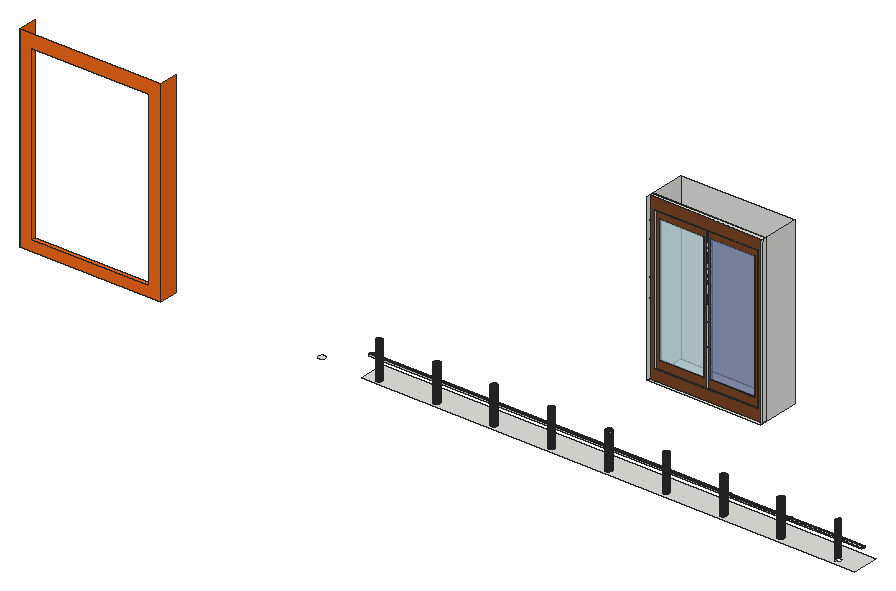
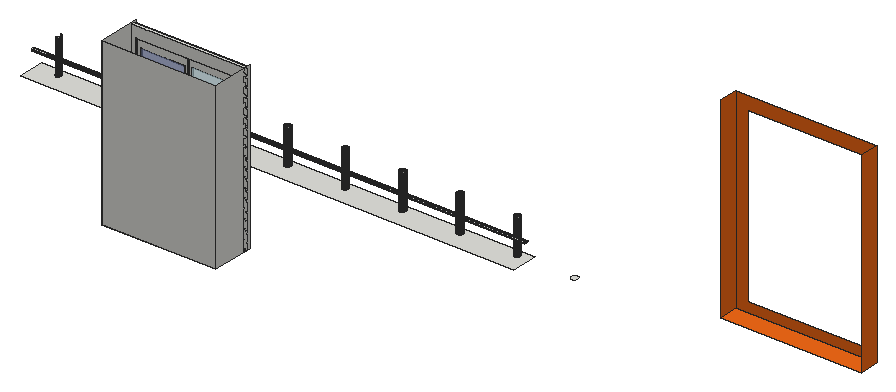
# SketchUp Ruby script. Lengths in inches.
U = 1.inch
M = Sketchup.active_model
def pt(a) = Geom::Point3d.new(a.map { |v| v * U })
def face(e, loops, mat)
  f = e.add_face(loops[0].map { |a| pt(a) })
  loops[1..].each { |l| e.add_face(l.map { |a| pt(a) }).erase! }
  f.material = f.back_material = mat if mat
  f
end
# faces: each face lists its corners as indices into pts; further lists are holes
def faces(e, pts, list, mat = nil) = list.each { |f| face(e, (f[0].is_a?(Array) ? f : [f]).map { |l| l.map { |i| pts[i] } }, mat) }
# xy, xz, yz: faces in a plane at the given z, y or x. An outline is a flat list of corners, or four numbers for a rectangle; further outlines are holes
def ring(l) = l.size == 4 ? [[l[0], l[1]], [l[2], l[1]], [l[2], l[3]], [l[0], l[3]]] : l.each_slice(2).to_a
def flat(e, list, mat, &to3) = list.each { |f| face(e, (f[0].is_a?(Array) ? f : [f]).map { |l| ring(l).map { |u, v| to3.(u, v) } }, mat) }
def xy(e, z, list, mat = nil) = flat(e, list, mat) { |x, y| [x, y, z] }
def xz(e, y, list, mat = nil) = flat(e, list, mat) { |x, z| [x, y, z] }
def yz(e, x, list, mat = nil) = flat(e, list, mat) { |y, z| [x, y, z] }
def lines(e, pts, list) = list.each { |a, b| e.add_line(pt(pts[a]), pt(pts[b])) }
# prism: a flat outline (further loops are holes) pulled along v
def prism(e, loops, v, mat = nil)
  f = face(e, loops, mat); d = Geom::Vector3d.new(v.map { |x| x * U })
  f.pushpull(f.normal.samedirection?(d) ? d.length : -d.length)
end
def box(e, o, s, mat = nil) = prism(e, [[o, [o[0] + s[0], o[1], o[2]], [o[0] + s[0], o[1] + s[1], o[2]], [o[0], o[1] + s[1], o[2]]]], [0, 0, s[2]], mat)
def at(x, y, z, deg = 0) = Geom::Transformation.translation(pt([x, y, z])) * Geom::Transformation.rotation(ORIGIN, Z_AXIS, deg.degrees)
def axes(o, x, y, z) = Geom::Transformation.new([*x, 0, *y, 0, *z, 0, *pt(o).to_a, 1])
def part(name) = M.definitions.add(name)
# library, detail: a bought-in or finely detailed component or shape, given as its bounding box
def library(name, o, s) = part(name).tap { |d| box(d.entities, o, s) }
def detail(e, o, s) = box(e.add_group.entities, o, s)
def put(e, d, t, mat = nil) = e.add_instance(d, t).tap { |i| i.material = mat if mat }
def group(e, t, mat = nil) = e.add_group.tap { |g| g.transformation = t; g.material = mat if mat }.entities
root = M.entities
M.materials.add("Generic").color = [243, 106, 23]
M.materials.add("[Translucent_Glass_Safety]").color = [204, 235, 244]
M.materials["[Translucent_Glass_Safety]"].alpha = 0.5
M.materials.add("[Translucent_Glass_Sky_Reflection]").color = [125, 138, 183]
M.materials["[Translucent_Glass_Sky_Reflection]"].alpha = 0.52
M.materials.add("[Wood Veneer 01]").color = [120, 70, 37]
c1 = part("Sliding window")
xy(c1.entities,0,[[0,0,4.33,55.51]])
xy(c1.entities,2.76,[[0,2.76,2,27.76],[3.15,2.76,4.33,27.76],[0,27.76,0.82,52.76],[0.82,27.76,2.36,52.76],[2.36,27.76,4.33,52.76]])
xy(c1.entities,4.72,[[2,4.72,2.4,26.38],[2.76,4.72,3.15,26.38],[0.82,29.13,1.22,50.79],[1.97,29.13,2.36,50.79]])
xy(c1.entities,36.61,[[2,4.72,2.4,26.38],[2.76,4.72,3.15,26.38],[0.82,29.13,1.22,50.79],[1.97,29.13,2.36,50.79]])
xy(c1.entities,38.58,[[0,2.76,2,27.76],[3.15,2.76,4.33,27.76],[0,27.76,0.82,52.76],[0.82,27.76,2.36,52.76],[2.36,27.76,4.33,52.76]])
xy(c1.entities,41.34,[[0,0,4.33,55.51]])
xz(c1.entities,0,[[0,0,4.33,41.34]])
xz(c1.entities,2.76,[[0,2.76,2,38.58],[3.15,2.76,4.33,38.58]])
xz(c1.entities,4.72,[[2,4.72,2.4,36.61],[2.76,4.72,3.15,36.61]])
xz(c1.entities,26.38,[[2,4.72,2.4,36.61],[2.76,4.72,3.15,36.61]])
xz(c1.entities,27.76,[[0.82,2.76,2,38.58],[2,2.76,2.36,38.58],[2.36,2.76,3.15,38.58]])
xz(c1.entities,29.13,[[0.82,4.72,1.22,36.61],[1.97,4.72,2.36,36.61]])
xz(c1.entities,50.79,[[0.82,4.72,1.22,36.61],[1.97,4.72,2.36,36.61]])
xz(c1.entities,52.76,[[0,2.76,0.82,38.58],[0.82,2.76,2.36,38.58],[2.36,2.76,4.33,38.58]])
xz(c1.entities,55.51,[[0,0,4.33,41.34]])
yz(c1.entities,0,[[[0,0,55.51,41.34],[2.76,2.76,52.76,38.58]]])
yz(c1.entities,0.82,[[[27.76,2.76,52.76,38.58],[29.13,4.72,50.79,36.61]]])
yz(c1.entities,1.22,[[29.13,4.72,50.79,36.61]],"[Translucent_Glass_Sky_Reflection]")
yz(c1.entities,1.97,[[29.13,4.72,50.79,36.61]],"[Translucent_Glass_Sky_Reflection]")
yz(c1.entities,2,[[[2.76,2.76,27.76,38.58],[4.72,4.72,26.38,36.61]]])
yz(c1.entities,2.36,[[[27.76,2.76,52.76,38.58],[29.13,4.72,50.79,36.61]]],"[Wood Veneer 01]")
yz(c1.entities,2.4,[[4.72,4.72,26.38,36.61]],"[Translucent_Glass_Safety]")
yz(c1.entities,2.76,[[4.72,4.72,26.38,36.61]],"[Translucent_Glass_Safety]")
yz(c1.entities,3.15,[[[2.76,2.76,27.76,38.58],[4.72,4.72,26.38,36.61]]],"[Wood Veneer 01]")
yz(c1.entities,4.33,[[[0,0,55.51,41.34],[2.76,2.76,52.76,38.58]]],"[Wood Veneer 01]")
xy(root,143.28,[[[220.54,127.4375,383.85,136.1875],[338.54,128.64,338.28,128.68,338.04,128.78,337.83,128.9375,337.67,129.14,337.57,129.39,337.54,129.64,337.57,129.9,337.67,130.14,337.83,130.35,338.04,130.51,338.28,130.61,338.54,130.64,338.79,130.61,339.04,130.51,339.24,130.35,339.4,130.14,339.5,129.9,339.54,129.64,339.5,129.39,339.4,129.14,339.24,128.9375,339.04,128.78,338.79,128.68],[319.54,128.64,319.28,128.68,319.04,128.78,318.83,128.9375,318.67,129.14,318.57,129.39,318.54,129.64,318.57,129.9,318.67,130.14,318.83,130.35,319.04,130.51,319.28,130.61,319.54,130.64,319.79,130.61,320.04,130.51,320.24,130.35,320.4,130.14,320.5,129.9,320.54,129.64,320.5,129.39,320.4,129.14,320.24,128.9375,320.04,128.78,319.79,128.68],[300.54,128.64,300.28,128.68,300.04,128.78,299.83,128.9375,299.67,129.14,299.57,129.39,299.54,129.64,299.57,129.9,299.67,130.14,299.83,130.35,300.04,130.51,300.28,130.61,300.54,130.64,300.79,130.61,301.04,130.51,301.24,130.35,301.4,130.14,301.5,129.9,301.54,129.64,301.5,129.39,301.4,129.14,301.24,128.9375,301.04,128.78,300.79,128.68],[281.54,128.64,281.28,128.68,281.04,128.78,280.83,128.9375,280.67,129.14,280.57,129.39,280.54,129.64,280.57,129.9,280.67,130.14,280.83,130.35,281.04,130.51,281.28,130.61,281.54,130.64,281.79,130.61,282.04,130.51,282.24,130.35,282.4,130.14,282.5,129.9,282.54,129.64,282.5,129.39,282.4,129.14,282.24,128.9375,282.04,128.78,281.79,128.68],[262.54,128.64,262.28,128.68,262.04,128.78,261.83,128.9375,261.67,129.14,261.57,129.39,261.54,129.64,261.57,129.9,261.67,130.14,261.83,130.35,262.04,130.51,262.28,130.61,262.54,130.64,262.79,130.61,263.04,130.51,263.24,130.35,263.4,130.14,263.5,129.9,263.54,129.64,263.5,129.39,263.4,129.14,263.24,128.9375,263.04,128.78,262.79,128.68],[243.54,128.64,243.28,128.68,243.04,128.78,242.83,128.9375,242.67,129.14,242.57,129.39,242.54,129.64,242.57,129.9,242.67,130.14,242.83,130.35,243.04,130.51,243.28,130.61,243.54,130.64,243.79,130.61,244.04,130.51,244.24,130.35,244.4,130.14,244.5,129.9,244.54,129.64,244.5,129.39,244.4,129.14,244.24,128.9375,244.04,128.78,243.79,128.68],[224.54,128.64,224.28,128.68,224.04,128.78,223.83,128.9375,223.67,129.14,223.57,129.39,223.54,129.64,223.57,129.9,223.67,130.14,223.83,130.35,224.04,130.51,224.28,130.61,224.54,130.64,224.79,130.61,225.04,130.51,225.24,130.35,225.4,130.14,225.5,129.9,225.54,129.64,225.5,129.39,225.4,129.14,225.24,128.9375,225.04,128.78,224.79,128.68],[376.66,128.64,376.4,128.68,376.16,128.78,375.95,128.9375,375.79,129.14,375.69,129.39,375.66,129.64,375.69,129.9,375.79,130.14,375.95,130.35,376.16,130.51,376.4,130.61,376.66,130.64,376.92,130.61,377.16,130.51,377.37,130.35,377.53,130.14,377.625,129.9,377.66,129.64,377.625,129.39,377.53,129.14,377.37,128.9375,377.16,128.78,376.92,128.68],[357.54,128.64,357.28,128.68,357.04,128.78,356.83,128.9375,356.67,129.14,356.57,129.39,356.54,129.64,356.57,129.9,356.67,130.14,356.83,130.35,357.04,130.51,357.28,130.61,357.54,130.64,357.79,130.61,358.04,130.51,358.24,130.35,358.4,130.14,358.5,129.9,358.54,129.64,358.5,129.39,358.4,129.14,358.24,128.9375,358.04,128.78,357.79,128.68]],[205.54,128.64,205.79,128.68,206.04,128.78,206.24,128.9375,206.4,129.14,206.5,129.39,206.54,129.64,206.5,129.9,206.4,130.14,206.24,130.35,206.04,130.51,205.79,130.61,205.54,130.64,205.28,130.61,205.04,130.51,204.83,130.35,204.67,130.14,204.57,129.9,204.54,129.64,204.57,129.39,204.67,129.14,204.83,128.9375,205.04,128.78,205.28,128.68]])
xy(root,144.25,[[279.74,171.4375,317.36,185.375]])
xy(root,146.92,[[112.41,121.25,158.88,127.4375]],"Generic")
xy(root,148.75,[[220.54,130.19,320.53,130.82],[320.53,130.19,338.84,130.82],[338.84,130.19,359.16,130.82],[359.16,130.19,378.85,130.82]])
xy(root,149.1875,[[220.54,130.19,320.53,130.82],[320.53,130.19,338.84,130.82],[338.84,130.19,383.85,130.82]])
xz(root,121.25,[[[112.41,146.92,158.88,211.52],[115.79,150.18,154.87,207.14]]],"Generic")
xz(root,130.19,[[220.54,148.75,383.85,149.1875]])
xz(root,130.82,[[220.54,149.0625,320.53,149.1875],[220.54,149.0625,320.53,149.1875],[320.53,149.0625,338.84,149.1875],[320.53,149.0625,338.84,149.1875],[338.84,149.0625,359.16,149.1875],
  [338.84,149.0625,359.16,149.1875],[359.16,149.0625,378.85,149.1875],[359.16,149.0625,378.85,149.1875]])
xz(root,131.35,[[220.54,148.72,383.85,149.04]])
xz(root,185.375,[[279.74,144.25,317.36,198.6875]])
yz(root,112.41,[[121.25,146.92,127.4375,211.52]],"Generic")
yz(root,158.88,[[121.25,146.92,127.4375,211.52]],"Generic")
yz(root,279.74,[[171.4375,144.25,185.375,198.6875]])
yz(root,317.36,[[171.4375,144.25,185.375,198.6875]])
p = [[224.28,128.68,143.28],[224.54,128.64,143.28],[224.54,128.64,155.04],[224.28,128.68,155.04],[224.79,128.68,143.28],[224.79,128.68,155.04],
  [243.28,128.68,143.28],[243.54,128.64,143.28],[243.54,128.64,155.04],[243.28,128.68,155.04],[243.79,128.68,143.28],[243.79,128.68,155.04],
  [262.28,128.68,143.28],[262.54,128.64,143.28],[262.54,128.64,155.04],[262.28,128.68,155.04],[262.79,128.68,143.28],[262.79,128.68,155.04],
  [281.28,128.68,143.28],[281.54,128.64,143.28],[281.54,128.64,155.04],[281.28,128.68,155.04],[281.79,128.68,143.28],[281.79,128.68,155.04],
  [300.28,128.68,143.28],[300.54,128.64,143.28],[300.54,128.64,155.04],[300.28,128.68,155.04],[300.79,128.68,143.28],[300.79,128.68,155.04],
  [319.28,128.68,143.28],[319.54,128.64,143.28],[319.54,128.64,155.04],[319.28,128.68,155.04],[319.79,128.68,143.28],[319.79,128.68,155.04],
  [338.28,128.68,143.28],[338.54,128.64,143.28],[338.54,128.64,155.04],[338.28,128.68,155.04],[338.79,128.68,143.28],[338.79,128.68,155.04],
  [357.28,128.68,143.28],[357.54,128.64,143.28],[357.54,128.64,155.04],[357.28,128.68,155.04],[357.79,128.68,143.28],[357.79,128.68,155.04],
  [224.04,128.78,143.28],[224.04,128.78,155.04],[225.04,128.78,143.28],[225.04,128.78,155.04],[243.04,128.78,143.28],[243.04,128.78,155.04],
  [244.04,128.78,143.28],[244.04,128.78,155.04],[262.04,128.78,143.28],[262.04,128.78,155.04],[263.04,128.78,143.28],[263.04,128.78,155.04],
  [281.04,128.78,143.28],[281.04,128.78,155.04],[282.04,128.78,143.28],[282.04,128.78,155.04],[300.04,128.78,143.28],[300.04,128.78,155.04],
  [301.04,128.78,143.28],[301.04,128.78,155.04],[319.04,128.78,143.28],[319.04,128.78,155.04],[320.04,128.78,143.28],[320.04,128.78,155.04],
  [338.04,128.78,143.28],[338.04,128.78,155.04],[339.04,128.78,143.28],[339.04,128.78,155.04],[357.04,128.78,143.28],[357.04,128.78,155.04],
  [358.04,128.78,143.28],[358.04,128.78,155.04],[376.16,128.78,143.28],[376.4,128.68,143.28],[376.4,128.68,155.04],[376.16,128.78,155.04],
  [223.83,128.9375,143.28],[223.83,128.9375,155.04],[225.24,128.9375,143.28],[225.24,128.9375,155.04],[242.83,128.9375,143.28],[242.83,128.9375,155.04],
  [244.24,128.9375,143.28],[244.24,128.9375,155.04],[261.83,128.9375,143.28],[261.83,128.9375,155.04],[263.24,128.9375,143.28],[263.24,128.9375,155.04],
  [280.83,128.9375,143.28],[280.83,128.9375,155.04],[282.24,128.9375,143.28],[282.24,128.9375,155.04],[299.83,128.9375,143.28],[299.83,128.9375,155.04],
  [301.24,128.9375,143.28],[301.24,128.9375,155.04],[318.83,128.9375,143.28],[318.83,128.9375,155.04],[320.24,128.9375,143.28],[320.24,128.9375,155.04],
  [337.83,128.9375,143.28],[337.83,128.9375,155.04],[339.24,128.9375,143.28],[339.24,128.9375,155.04],[356.83,128.9375,143.28],[356.83,128.9375,155.04],
  [358.24,128.9375,143.28],[358.24,128.9375,155.04],[375.95,128.9375,143.28],[375.95,128.9375,155.04],[223.67,129.14,143.28],[223.67,129.14,155.04],
  [225.4,129.14,143.28],[225.4,129.14,155.04],[242.67,129.14,143.28],[242.67,129.14,155.04],[244.4,129.14,143.28],[244.4,129.14,155.04],
  [261.67,129.14,143.28],[261.67,129.14,155.04],[263.4,129.14,143.28],[263.4,129.14,155.04],[280.67,129.14,143.28],[280.67,129.14,155.04],
  [282.4,129.14,143.28],[282.4,129.14,155.04],[299.67,129.14,143.28],[299.67,129.14,155.04],[301.4,129.14,143.28],[301.4,129.14,155.04],
  [318.67,129.14,143.28],[318.67,129.14,155.04],[320.4,129.14,143.28],[320.4,129.14,155.04],[337.67,129.14,143.28],[337.67,129.14,155.04],
  [339.4,129.14,143.28],[339.4,129.14,155.04],[356.67,129.14,143.28],[356.67,129.14,155.04],[358.4,129.14,143.28],[358.4,129.14,155.04],
  [375.79,129.14,143.28],[375.79,129.14,155.04],[223.57,129.39,143.28],[223.57,129.39,155.04],[225.5,129.39,143.28],[225.5,129.39,155.04],
  [242.57,129.39,143.28],[242.57,129.39,155.04],[244.5,129.39,143.28],[244.5,129.39,155.04],[261.57,129.39,143.28],[261.57,129.39,155.04],
  [263.5,129.39,143.28],[263.5,129.39,155.04],[280.57,129.39,143.28],[280.57,129.39,155.04],[282.5,129.39,143.28],[282.5,129.39,155.04],
  [299.57,129.39,143.28],[299.57,129.39,155.04],[301.5,129.39,143.28],[301.5,129.39,155.04],[318.57,129.39,143.28],[318.57,129.39,155.04],
  [320.5,129.39,143.28],[320.5,129.39,155.04],[337.57,129.39,143.28],[337.57,129.39,155.04],[339.5,129.39,143.28],[339.5,129.39,155.04],
  [356.57,129.39,143.28],[356.57,129.39,155.04],[358.5,129.39,143.28],[358.5,129.39,155.04],[375.69,129.39,143.28],[375.69,129.39,155.04],
  [223.54,129.64,143.28],[223.54,129.64,155.04],[225.54,129.64,143.28],[225.54,129.64,155.04],[242.54,129.64,143.28],[242.54,129.64,155.04],
  [244.54,129.64,143.28],[244.54,129.64,155.04],[261.54,129.64,143.28],[261.54,129.64,155.04],[263.54,129.64,143.28],[263.54,129.64,155.04],
  [280.54,129.64,143.28],[280.54,129.64,155.04],[282.54,129.64,143.28],[282.54,129.64,155.04],[299.54,129.64,143.28],[299.54,129.64,155.04],
  [301.54,129.64,143.28],[301.54,129.64,155.04],[318.54,129.64,143.28],[318.54,129.64,155.04],[320.54,129.64,143.28],[320.54,129.64,155.04],
  [337.54,129.64,143.28],[337.54,129.64,155.04],[339.54,129.64,143.28],[339.54,129.64,155.04],[356.54,129.64,143.28],[356.54,129.64,155.04],
  [358.54,129.64,143.28],[358.54,129.64,155.04],[375.66,129.64,143.28],[375.66,129.64,155.04],[223.57,129.9,143.28],[223.57,129.9,155.04],
  [225.5,129.9,143.28],[225.5,129.9,155.04],[242.57,129.9,143.28],[242.57,129.9,155.04],[244.5,129.9,143.28],[244.5,129.9,155.04],
  [261.57,129.9,143.28],[261.57,129.9,155.04],[263.5,129.9,143.28],[263.5,129.9,155.04],[280.57,129.9,143.28],[280.57,129.9,155.04],
  [282.5,129.9,143.28],[282.5,129.9,155.04],[299.57,129.9,143.28],[299.57,129.9,155.04],[301.5,129.9,143.28],[301.5,129.9,155.04],
  [318.57,129.9,143.28],[318.57,129.9,155.04],[320.5,129.9,143.28],[320.5,129.9,155.04],[337.57,129.9,143.28],[337.57,129.9,155.04],
  [339.5,129.9,143.28],[339.5,129.9,155.04],[356.57,129.9,143.28],[356.57,129.9,155.04],[358.5,129.9,143.28],[358.5,129.9,155.04],
  [375.69,129.9,143.28],[375.69,129.9,155.04],[223.67,130.14,143.28],[223.67,130.14,155.04],[225.4,130.14,143.28],[225.4,130.14,155.04],
  [242.67,130.14,143.28],[242.67,130.14,155.04],[244.4,130.14,143.28],[244.4,130.14,155.04],[261.67,130.14,143.28],[261.67,130.14,155.04],
  [263.4,130.14,143.28],[263.4,130.14,155.04],[280.67,130.14,143.28],[280.67,130.14,155.04],[282.4,130.14,143.28],[282.4,130.14,155.04],
  [299.67,130.14,143.28],[299.67,130.14,155.04],[301.4,130.14,143.28],[301.4,130.14,155.04],[318.67,130.14,143.28],[318.67,130.14,155.04],
  [320.4,130.14,143.28],[320.4,130.14,155.04],[337.67,130.14,143.28],[337.67,130.14,155.04],[339.4,130.14,143.28],[339.4,130.14,155.04],
  [356.67,130.14,143.28],[356.67,130.14,155.04],[358.4,130.14,143.28],[358.4,130.14,155.04],[375.79,130.14,143.28],[375.79,130.14,155.04],
  [223.83,130.35,143.28],[223.83,130.35,155.04],[225.24,130.35,143.28],[225.24,130.35,155.04],[242.83,130.35,143.28],[242.83,130.35,155.04],
  [244.24,130.35,143.28],[244.24,130.35,155.04],[261.83,130.35,143.28],[261.83,130.35,155.04],[263.24,130.35,143.28],[263.24,130.35,155.04],
  [280.83,130.35,143.28],[280.83,130.35,155.04],[282.24,130.35,143.28],[282.24,130.35,155.04],[299.83,130.35,143.28],[299.83,130.35,155.04],
  [301.24,130.35,143.28],[301.24,130.35,155.04],[318.83,130.35,143.28],[318.83,130.35,155.04],[320.24,130.35,143.28],[320.24,130.35,155.04],
  [337.83,130.35,143.28],[337.83,130.35,155.04],[339.24,130.35,143.28],[339.24,130.35,155.04],[356.83,130.35,143.28],[356.83,130.35,155.04],
  [358.24,130.35,143.28],[358.24,130.35,155.04],[375.95,130.35,143.28],[375.95,130.35,155.04],[224.04,130.51,143.28],[224.04,130.51,155.04],
  [225.04,130.51,143.28],[225.04,130.51,155.04],[243.04,130.51,143.28],[243.04,130.51,155.04],[244.04,130.51,143.28],[244.04,130.51,155.04],
  [262.04,130.51,143.28],[262.04,130.51,155.04],[263.04,130.51,143.28],[263.04,130.51,155.04],[281.04,130.51,143.28],[281.04,130.51,155.04],
  [282.04,130.51,143.28],[282.04,130.51,155.04],[300.04,130.51,143.28],[300.04,130.51,155.04],[301.04,130.51,143.28],[301.04,130.51,155.04],
  [319.04,130.51,143.28],[319.04,130.51,155.04],[320.04,130.51,143.28],[320.04,130.51,155.04],[338.04,130.51,143.28],[338.04,130.51,155.04],
  [339.04,130.51,143.28],[339.04,130.51,155.04],[357.04,130.51,143.28],[357.04,130.51,155.04],[358.04,130.51,143.28],[358.04,130.51,155.04],
  [376.16,130.51,143.28],[376.16,130.51,155.04],[224.28,130.61,143.28],[224.28,130.61,155.04],[224.79,130.61,143.28],[224.79,130.61,155.04],
  [243.28,130.61,143.28],[243.28,130.61,155.04],[243.79,130.61,143.28],[243.79,130.61,155.04],[262.28,130.61,143.28],[262.28,130.61,155.04],
  [262.79,130.61,143.28],[262.79,130.61,155.04],[281.28,130.61,143.28],[281.28,130.61,155.04],[281.79,130.61,143.28],[281.79,130.61,155.04],
  [300.28,130.61,143.28],[300.28,130.61,155.04],[300.79,130.61,143.28],[300.79,130.61,155.04],[319.28,130.61,143.28],[319.28,130.61,155.04],
  [319.79,130.61,143.28],[319.79,130.61,155.04],[338.28,130.61,143.28],[338.28,130.61,155.04],[338.79,130.61,143.28],[338.79,130.61,155.04],
  [357.28,130.61,143.28],[357.28,130.61,155.04],[357.79,130.61,143.28],[357.79,130.61,155.04],[376.4,130.61,143.28],[376.4,130.61,155.04],
  [224.54,130.64,143.28],[224.54,130.64,155.04],[243.54,130.64,143.28],[243.54,130.64,155.04],[262.54,130.64,143.28],[262.54,130.64,155.04],
  [281.54,130.64,143.28],[281.54,130.64,155.04],[300.54,130.64,143.28],[300.54,130.64,155.04],[319.54,130.64,143.28],[319.54,130.64,155.04],
  [338.54,130.64,143.28],[338.54,130.64,155.04],[357.54,130.64,143.28],[357.54,130.64,155.04],[376.66,130.64,143.28],[376.66,130.64,155.04],
  [338.84,130.82,148.75],[320.53,130.82,148.75],[220.54,130.82,148.75],[220.54,131.35,148.72],[320.53,131.35,148.72],[338.84,131.35,148.72],
  [359.16,131.35,148.72],[378.85,131.35,148.72],[383.85,131.35,148.72],[383.85,130.82,148.75],[378.85,130.82,148.75],[359.16,130.82,148.75],
  [320.53,131.35,149.04],[220.54,131.35,149.04],[220.54,131.36,149.16],[320.53,131.36,149.16],[338.84,131.35,149.04],[338.84,131.36,149.16],
  [359.16,131.35,149.04],[359.16,131.36,149.16],[378.85,131.35,149.04],[378.85,131.36,149.16],[220.54,130.82,149.1875],[320.53,130.82,149.1875],
  [338.84,130.82,149.1875],[359.16,130.82,149.1875],[378.85,130.82,149.1875],[383.85,130.82,149.1875],[383.85,131.36,149.16],[357.54,129.64,143.28],
  [357.54,129.64,155.47],[338.41,129.64,143.28],[338.41,129.64,155.47],[319.29,129.64,143.28],[319.29,129.64,155.47],[300.16,129.64,143.28],
  [300.16,129.64,155.47],[281.04,129.64,143.28],[281.04,129.64,155.47],[261.91,129.64,143.28],[261.91,129.64,155.47],[242.79,129.64,143.28],
  [242.79,129.64,155.47],[223.66,129.64,143.28],[223.66,129.64,155.47],[359.16,130.96,148.9],[338.84,130.96,148.9],[378.85,130.96,148.9],
  [320.53,130.96,148.9],[220.54,130.96,148.9]]
faces(root,p,[[0,1,2,3],[1,4,5,2],[6,7,8,9],[7,10,11,8],[12,13,14,15],[13,16,17,14],[18,19,20,21],[19,22,23,20],
  [24,25,26,27],[25,28,29,26],[30,31,32,33],[31,34,35,32],[36,37,38,39],[37,40,41,38],[42,43,44,45],[43,46,47,44],
  [48,0,3,49],[4,50,51,5],[52,6,9,53],[10,54,55,11],[56,12,15,57],[16,58,59,17],[60,18,21,61],[22,62,63,23],
  [64,24,27,65],[28,66,67,29],[68,30,33,69],[34,70,71,35],[72,36,39,73],[40,74,75,41],[76,42,45,77],[46,78,79,47],
  [80,81,82,83],[84,48,49,85],[50,86,87,51],[88,52,53,89],[54,90,91,55],[92,56,57,93],[58,94,95,59],[96,60,61,97],
  [62,98,99,63],[100,64,65,101],[66,102,103,67],[104,68,69,105],[70,106,107,71],[108,72,73,109],[74,110,111,75],[112,76,77,113],
  [78,114,115,79],[116,80,83,117],[118,84,85,119],[86,120,121,87],[122,88,89,123],[90,124,125,91],[126,92,93,127],[94,128,129,95],
  [130,96,97,131],[98,132,133,99],[134,100,101,135],[102,136,137,103],[138,104,105,139],[106,140,141,107],[142,108,109,143],[110,144,145,111],
  [146,112,113,147],[114,148,149,115],[150,116,117,151],[152,118,119,153],[120,154,155,121],[156,122,123,157],[124,158,159,125],[160,126,127,161],
  [128,162,163,129],[164,130,131,165],[132,166,167,133],[168,134,135,169],[136,170,171,137],[172,138,139,173],[140,174,175,141],[176,142,143,177],
  [144,178,179,145],[180,146,147,181],[148,182,183,149],[184,150,151,185],[186,152,153,187],[154,188,189,155],[190,156,157,191],[158,192,193,159],
  [194,160,161,195],[162,196,197,163],[198,164,165,199],[166,200,201,167],[202,168,169,203],[170,204,205,171],[206,172,173,207],[174,208,209,175],
  [210,176,177,211],[178,212,213,179],[214,180,181,215],[182,216,217,183],[218,184,185,219],[220,186,187,221],[188,222,223,189],[224,190,191,225],
  [192,226,227,193],[228,194,195,229],[196,230,231,197],[232,198,199,233],[200,234,235,201],[236,202,203,237],[204,238,239,205],[240,206,207,241],
  [208,242,243,209],[244,210,211,245],[212,246,247,213],[248,214,215,249],[216,250,251,217],[252,218,219,253],[254,220,221,255],[222,256,257,223],
  [258,224,225,259],[226,260,261,227],[262,228,229,263],[230,264,265,231],[266,232,233,267],[234,268,269,235],[270,236,237,271],[238,272,273,239],
  [274,240,241,275],[242,276,277,243],[278,244,245,279],[246,280,281,247],[282,248,249,283],[250,284,285,251],[286,252,253,287],[288,254,255,289],
  [256,290,291,257],[292,258,259,293],[260,294,295,261],[296,262,263,297],[264,298,299,265],[300,266,267,301],[268,302,303,269],[304,270,271,305],
  [272,306,307,273],[308,274,275,309],[276,310,311,277],[312,278,279,313],[280,314,315,281],[316,282,283,317],[284,318,319,285],[320,286,287,321],
  [322,288,289,323],[290,324,325,291],[326,292,293,327],[294,328,329,295],[330,296,297,331],[298,332,333,299],[334,300,301,335],[302,336,337,303],
  [338,304,305,339],[306,340,341,307],[342,308,309,343],[310,344,345,311],[346,312,313,347],[314,348,349,315],[350,316,317,351],[318,352,353,319],
  [354,320,321,355],[356,322,323,357],[324,358,359,325],[360,326,327,361],[328,362,363,329],[364,330,331,365],[332,366,367,333],[368,334,335,369],
  [336,370,371,337],[372,338,339,373],[340,374,375,341],[376,342,343,377],[344,378,379,345],[380,346,347,381],[348,382,383,349],[384,350,351,385],
  [352,386,387,353],[388,354,355,389],[390,356,357,391],[358,390,391,359],[392,360,361,393],[362,392,393,363],[394,364,365,395],[366,394,395,367],
  [396,368,369,397],[370,396,397,371],[398,372,373,399],[374,398,399,375],[400,376,377,401],[378,400,401,379],[402,380,381,403],[382,402,403,383],
  [404,384,385,405],[386,404,405,387],[406,388,389,407],[408,409,410,411,412,413,414,415,416,417,418,419],[420,421,422,423],[424,420,423,425],[426,424,425,427],[428,426,427,429],
  [429,427,425,423,422,430,431,432,433,434,435,436]])
lines(root,p,[[437,438],[439,440],[441,442],[443,444],[445,446],[447,448],[449,450],[451,452],[453,454],[455,453],[456,457],[454,456]])
put(root,c1,axes([279.74,173.65,144.25],[0,-0.28,0],[0.67778,0,0],[0,0,1.31687]))
